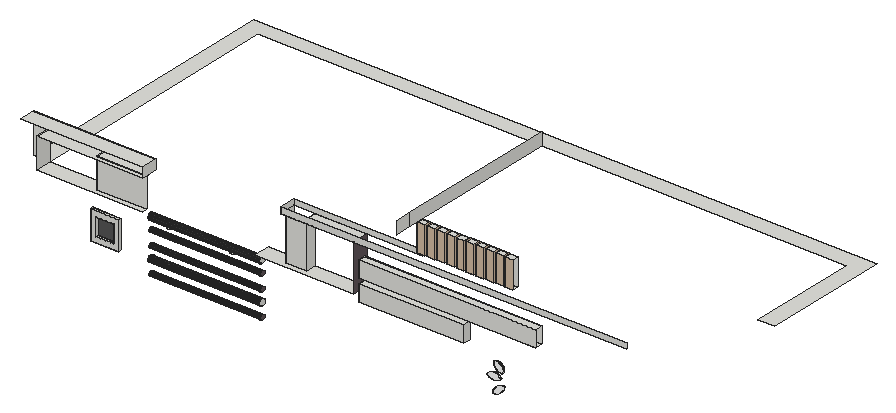
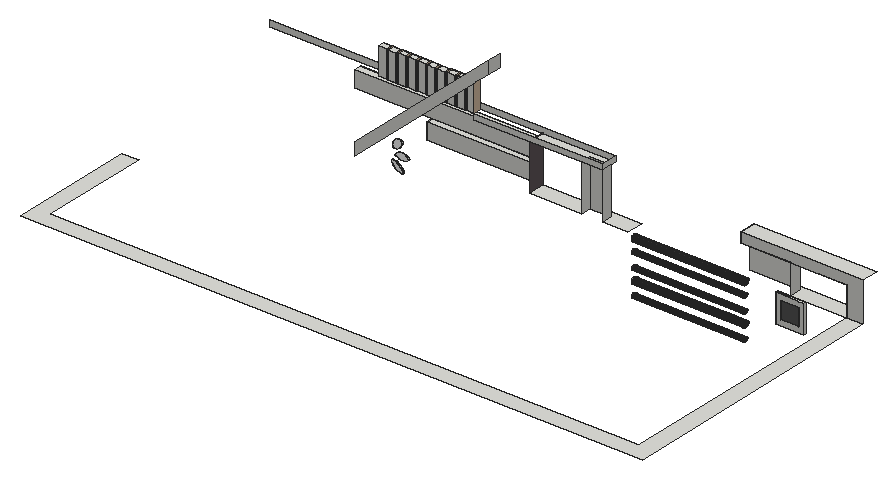
# SketchUp Ruby script. Lengths in inches.
U = 1.inch
M = Sketchup.active_model
def pt(a) = Geom::Point3d.new(a.map { |v| v * U })
def face(e, loops, mat)
  f = e.add_face(loops[0].map { |a| pt(a) })
  loops[1..].each { |l| e.add_face(l.map { |a| pt(a) }).erase! }
  f.material = f.back_material = mat if mat
  f
end
# faces: each face lists its corners as indices into pts; further lists are holes
def faces(e, pts, list, mat = nil) = list.each { |f| face(e, (f[0].is_a?(Array) ? f : [f]).map { |l| l.map { |i| pts[i] } }, mat) }
# xy, xz, yz: faces in a plane at the given z, y or x. An outline is a flat list of corners, or four numbers for a rectangle; further outlines are holes
def ring(l) = l.size == 4 ? [[l[0], l[1]], [l[2], l[1]], [l[2], l[3]], [l[0], l[3]]] : l.each_slice(2).to_a
def flat(e, list, mat, &to3) = list.each { |f| face(e, (f[0].is_a?(Array) ? f : [f]).map { |l| ring(l).map { |u, v| to3.(u, v) } }, mat) }
def xy(e, z, list, mat = nil) = flat(e, list, mat) { |x, y| [x, y, z] }
def xz(e, y, list, mat = nil) = flat(e, list, mat) { |x, z| [x, y, z] }
def yz(e, x, list, mat = nil) = flat(e, list, mat) { |y, z| [x, y, z] }
def lines(e, pts, list) = list.each { |a, b| e.add_line(pt(pts[a]), pt(pts[b])) }
# prism: a flat outline (further loops are holes) pulled along v
def prism(e, loops, v, mat = nil)
  f = face(e, loops, mat); d = Geom::Vector3d.new(v.map { |x| x * U })
  f.pushpull(f.normal.samedirection?(d) ? d.length : -d.length)
end
def box(e, o, s, mat = nil) = prism(e, [[o, [o[0] + s[0], o[1], o[2]], [o[0] + s[0], o[1] + s[1], o[2]], [o[0], o[1] + s[1], o[2]]]], [0, 0, s[2]], mat)
def at(x, y, z, deg = 0) = Geom::Transformation.translation(pt([x, y, z])) * Geom::Transformation.rotation(ORIGIN, Z_AXIS, deg.degrees)
def axes(o, x, y, z) = Geom::Transformation.new([*x, 0, *y, 0, *z, 0, *pt(o).to_a, 1])
def part(name) = M.definitions.add(name)
# library, detail: a bought-in or finely detailed component or shape, given as its bounding box
def library(name, o, s) = part(name).tap { |d| box(d.entities, o, s) }
def detail(e, o, s) = box(e.add_group.entities, o, s)
def put(e, d, t, mat = nil) = e.add_instance(d, t).tap { |i| i.material = mat if mat }
def group(e, t, mat = nil) = e.add_group.tap { |g| g.transformation = t; g.material = mat if mat }.entities
root = M.entities
M.materials.add("[Asphalt New]").color = [96, 86, 89]
M.materials.add("[Color M00]").color = [255, 255, 255]
M.materials.add("[Color M06]").color = [86, 86, 86]
M.materials.add("[Color M07]").color = [58, 58, 58]
M.materials.add("[Formica Laminate Light]").color = [213, 189, 164]
box(root,[255.42,148.16,262.6875],[57.81,4.19,8.9375])
prism(root,[[[323.7,152.35,248.91],[323.08,152.35,249.43],[323.52,152.35,249.97],[324.07,152.35,250.4375],[324.71,152.35,250.82],[325.41,152.35,251.1],[326.17,152.35,251.27],[326.94,152.35,251.33],[327.72,152.35,251.27],[328.47,152.35,251.1],[329.18,152.35,250.82],[329.8125,152.35,250.4375],[330.36,152.35,249.97],[330.81,152.35,249.43],[330.18,152.35,248.91],[329.46,152.35,248.49],[328.66,152.35,248.18],[327.82,152.35,247.99],[326.94,152.35,247.92],[326.07,152.35,247.99],[325.22,152.35,248.18],[324.43,152.35,248.49]]],[0,-0.5625,0],"[Color M00]")
xy(root,239.3,[[105.86,150.85,121.54,152.35]])
xy(root,242.21,[[108.76,150.85,118.64,152.35]])
xy(root,252.08,[[108.76,150.85,118.64,152.35]])
xy(root,254.99,[[105.86,150.85,121.54,152.35]])
xy(root,257.37,[[145.55,154.65,145.96,154.7,146.33,154.86,146.66,155.11,146.9,155.43,147.0625,155.81,147.08,155.94,144.02,155.94,144.04,155.81,144.2,155.43,144.45,155.11,144.77,154.86,145.15,154.7],[180.11,154.65,180.52,154.7,180.9,154.86,181.22,155.11,181.47,155.43,181.625,155.81,181.64,155.94,178.59,155.94,178.6,155.81,178.76,155.43,179.01,155.11,179.33,154.86,179.71,154.7],[144.02,155.94,147.08,155.94,147.11,156.21,147.0625,156.62,146.9,156.99,146.66,157.32,146.33,157.57,145.96,157.72,145.55,157.77,145.15,157.72,144.77,157.57,144.45,157.32,144.2,156.99,144.04,156.62,143.99,156.21],[178.59,155.94,181.64,155.94,181.68,156.21,181.625,156.62,181.47,156.99,181.22,157.32,180.9,157.57,180.52,157.72,180.11,157.77,179.71,157.72,179.33,157.57,179.01,157.32,178.76,156.99,178.6,156.62,178.55,156.21]])
xy(root,262.6875,[[74.99,152.35,133.58,152.35,133.58,154.79,106.04,154.79,106.04,161.35,74.99,161.35],[195.29,152.35,249.72,152.35,249.72,161.35,220.78,161.35,220.78,155.66,209.34,155.66,209.34,161.35,195.29,161.35],[65.99,161.35,74.99,161.35,74.99,304.28,399.27,304.28,399.27,243.33,408.27,243.33,408.27,313.28,65.99,313.28]])
xy(root,274.4,[[255.42,148.16,353.17,152.35]])
xy(root,279.1,[[74.99,152.35,133.58,161.35]])
xy(root,279.1875,[[106.04,154.79,133.58,161.35]])
xy(root,283.34,[[255.42,148.16,353.17,152.35]])
xy(root,284.4375,[[65.99,152.35,133.58,161.35]])
xy(root,288.3125,[[209.34,152.35,209.34,155.66,220.78,155.66,220.78,161.35,249.72,161.35,249.72,152.35]])
xy(root,291.4375,[[280.02,157.85,284.38,161.35],[285.39,157.85,289.76,161.35],[290.77,157.85,295.13,161.35],[296.14,157.85,300.51,161.35],[301.52,157.85,305.88,161.35],
  [306.89,157.85,311.26,161.35],[312.27,157.85,316.63,161.35],[317.64,157.85,322.01,161.35],[323.02,157.85,327.38,161.35],[328.39,157.85,332.76,161.35]])
xy(root,306.375,[[280.02,157.85,284.38,161.35],[285.39,157.85,289.76,161.35],[290.77,157.85,295.13,161.35],[296.14,157.85,300.51,161.35],[301.52,157.85,305.88,161.35],
  [306.89,157.85,311.26,161.35],[312.27,157.85,316.63,161.35],[317.64,157.85,322.01,161.35],[323.02,157.85,327.38,161.35],[328.39,157.85,332.76,161.35]])
xz(root,148.16,[[255.42,274.4,353.17,283.34]])
xz(root,150.85,[[[105.86,239.3,121.54,254.99],[108.76,242.21,118.64,252.08]]])
xz(root,151.79,[[326.99,241.29,327.73,241.32,328.46,241.46,329.16,241.68,329.83,242,330.45,242.4,331.01,242.89,331.5,243.4375,331.92,244.05,332.25,244.71,332.5,245.4,332.64,246.13,331.92,246.15,331.19,246.09,330.48,245.93,329.79,245.69,329.14,245.37,328.53,244.97,327.97,244.5,327.48,243.96,327.05,243.37,326.7,242.73,326.4375,242.06,326.25,241.35],[331.37,252.53,332.01,252.625,332.1875,253.33,332.22,254.0625,332.1,254.78,331.84,255.47,331.45,256.08,330.9375,256.6,330.33,257.01,329.66,257.29,328.94,257.43,328.21,257.42,327.5,257.27,326.83,256.97,326.85,256.32,326.97,255.68,327.1875,255.07,327.5,254.5,327.89,253.98,328.35,253.52,328.88,253.14,329.46,252.85,330.08,252.65,330.72,252.54]],"[Color M00]")
xz(root,152.35,[[[105.86,239.3,121.54,254.99],[108.76,242.21,118.64,252.08]],[255.42,274.4,353.17,283.34],[209.34,288.3125,399.65,291.4375]])
xz(root,152.35,[[326.99,241.29,326.25,241.35,326.4375,242.06,326.7,242.73,327.05,243.37,327.48,243.96,327.97,244.5,328.53,244.97,329.14,245.37,329.79,245.69,330.48,245.93,331.19,246.09,331.92,246.15,332.64,246.13,332.5,245.4,332.25,244.71,331.92,244.05,331.5,243.4375,331.01,242.89,330.45,242.4,329.83,242,329.16,241.68,328.46,241.46,327.73,241.32],[331.37,252.53,330.72,252.54,330.08,252.65,329.46,252.85,328.88,253.14,328.35,253.52,327.89,253.98,327.5,254.5,327.1875,255.07,326.97,255.68,326.85,256.32,326.83,256.97,327.5,257.27,328.21,257.42,328.94,257.43,329.66,257.29,330.33,257.01,330.9375,256.6,331.45,256.08,331.84,255.47,332.1,254.78,332.22,254.0625,332.1875,253.33,332.01,252.625]],"[Color M00]")
xz(root,152.35,[[108.76,242.21,118.64,252.08]],"[Color M06]")
xz(root,154.79,[[106.04,262.6875,133.58,279.1875]])
xz(root,155.66,[[209.34,262.6875,220.78,288.3125]])
xz(root,157.85,[[280.02,291.4375,284.38,306.375],[285.39,291.4375,289.76,306.375],[290.77,291.4375,295.13,306.375],[296.14,291.4375,300.51,306.375],[301.52,291.4375,305.88,306.375],
  [306.89,291.4375,311.26,306.375],[312.27,291.4375,316.63,306.375],[317.64,291.4375,322.01,306.375],[323.02,291.4375,327.38,306.375],[328.39,291.4375,332.76,306.375]],"[Formica Laminate Light]")
xz(root,161.35,[[65.99,262.6875,65.99,284.4375,133.58,284.4375,133.58,279.1875,106.04,279.1875,106.04,279.1,74.99,279.1,74.99,262.6875],[106.04,279.1,133.58,279.1875],[209.34,288.3125,280.02,291.4375],[280.02,291.4375,284.38,306.375],[284.38,291.4375,285.39,306.375],
  [285.39,291.4375,289.76,306.375],[289.76,291.4375,290.77,306.375],[290.77,291.4375,295.13,306.375],[295.13,291.4375,296.14,306.375],[296.14,291.4375,300.51,306.375],
  [300.51,291.4375,301.52,306.375],[301.52,291.4375,305.88,306.375],[305.88,291.4375,306.89,306.375],[306.89,291.4375,311.26,306.375],[311.26,291.4375,312.27,306.375],
  [312.27,291.4375,316.63,306.375],[316.63,291.4375,317.64,306.375],[317.64,291.4375,322.01,306.375],[322.01,291.4375,323.02,306.375],[323.02,291.4375,327.38,306.375],
  [327.38,291.4375,328.39,306.375],[328.39,291.4375,332.76,306.375]])
yz(root,74.99,[[152.35,262.6875,161.35,279.1]])
yz(root,105.86,[[150.85,239.3,152.35,254.99]])
yz(root,106.04,[[154.79,262.6875,161.35,279.1875]])
yz(root,108.76,[[150.85,242.21,152.35,252.08]])
yz(root,118.64,[[150.85,242.21,152.35,252.08]])
yz(root,121.54,[[150.85,239.3,152.35,254.99]])
yz(root,133.58,[[152.35,279.1,154.79,279.1,154.79,279.1875,161.35,279.1875,161.35,284.4375,152.35,284.4375],[154.79,279.1,161.35,279.1875]])
yz(root,195.29,[[157.4,235.59,157.84,235.65,158.25,235.82,158.6,236.08,158.87,236.43,159.03,236.84,159.09,237.28,159.03,237.71,158.87,238.12,158.6,238.47,158.25,238.74,157.84,238.91,157.4,238.96,156.97,238.91,156.5625,238.74,156.21,238.47,155.94,238.12,155.77,237.71,155.72,237.28,155.77,236.84,155.94,236.43,156.21,236.08,156.5625,235.82,156.97,235.65],[157.4,256.53,157.84,256.58,158.25,256.75,158.6,257.02,158.87,257.37,159.03,257.78,159.09,258.21,159.03,258.65,158.87,259.06,158.6,259.41,158.25,259.68,157.84,259.84,157.4,259.9,156.97,259.84,156.5625,259.68,156.21,259.41,155.94,259.06,155.77,258.65,155.72,258.21,155.77,257.78,155.94,257.37,156.21,257.02,156.5625,256.75,156.97,256.58]])
yz(root,195.29,[[157.64,228.69,157.94,228.73,158.23,228.85,158.48,229.04,158.67,229.28,158.78,229.57,158.82,229.88,158.78,230.1875,158.67,230.47,158.48,230.72,158.23,230.91,157.94,231.03,157.64,231.07,157.33,231.03,157.04,230.91,156.8,230.72,156.61,230.47,156.49,230.1875,156.45,229.88,156.49,229.57,156.61,229.28,156.8,229.04,157.04,228.85,157.33,228.73],[157.64,242.44,157.94,242.48,158.23,242.6,158.48,242.79,158.67,243.03,158.78,243.32,158.82,243.63,158.78,243.9375,158.67,244.22,158.48,244.47,158.23,244.66,157.94,244.78,157.64,244.82,157.33,244.78,157.04,244.66,156.8,244.47,156.61,244.22,156.49,243.9375,156.45,243.63,156.49,243.32,156.61,243.03,156.8,242.79,157.04,242.6,157.33,242.48],[157.64,250.38,157.94,250.42,158.23,250.54,158.48,250.73,158.67,250.97,158.78,251.26,158.82,251.57,158.78,251.875,158.67,252.16,158.48,252.41,158.23,252.59,157.94,252.71,157.64,252.75,157.33,252.71,157.04,252.59,156.8,252.41,156.61,252.16,156.49,251.875,156.45,251.57,156.49,251.26,156.61,250.97,156.8,250.73,157.04,250.54,157.33,250.42]],"[Asphalt New]")
yz(root,209.34,[[155.66,262.6875,161.35,288.3125],[152.35,288.3125,161.35,291.4375]])
yz(root,220.78,[[155.66,262.6875,161.35,288.3125]])
yz(root,249.72,[[152.35,262.6875,161.35,288.3125]],"[Asphalt New]")
yz(root,255.42,[[148.16,274.4,152.35,283.34]])
yz(root,280.02,[[143.85,306.375,152.35,313.1875],[152.35,306.375,243.33,313.1875]])
yz(root,280.02,[[157.85,291.4375,161.35,306.375]],"[Formica Laminate Light]")
yz(root,284.38,[[157.85,291.4375,161.35,306.375]],"[Formica Laminate Light]")
yz(root,285.39,[[157.85,291.4375,161.35,306.375]],"[Formica Laminate Light]")
yz(root,289.76,[[157.85,291.4375,161.35,306.375]],"[Formica Laminate Light]")
yz(root,290.77,[[157.85,291.4375,161.35,306.375]],"[Formica Laminate Light]")
yz(root,295.13,[[157.85,291.4375,161.35,306.375]],"[Formica Laminate Light]")
yz(root,296.14,[[157.85,291.4375,161.35,306.375]],"[Formica Laminate Light]")
yz(root,300.51,[[157.85,291.4375,161.35,306.375]],"[Formica Laminate Light]")
yz(root,301.52,[[157.85,291.4375,161.35,306.375]],"[Formica Laminate Light]")
yz(root,305.88,[[157.85,291.4375,161.35,306.375]],"[Formica Laminate Light]")
yz(root,306.89,[[157.85,291.4375,161.35,306.375]],"[Formica Laminate Light]")
yz(root,311.26,[[157.85,291.4375,161.35,306.375]],"[Formica Laminate Light]")
yz(root,312.27,[[157.85,291.4375,161.35,306.375]],"[Formica Laminate Light]")
yz(root,316.63,[[157.85,291.4375,161.35,306.375]],"[Formica Laminate Light]")
yz(root,317.64,[[157.85,291.4375,161.35,306.375]],"[Formica Laminate Light]")
yz(root,322.01,[[157.85,291.4375,161.35,306.375]],"[Formica Laminate Light]")
yz(root,323.02,[[157.85,291.4375,161.35,306.375]],"[Formica Laminate Light]")
yz(root,327.38,[[157.85,291.4375,161.35,306.375]],"[Formica Laminate Light]")
yz(root,328.39,[[157.85,291.4375,161.35,306.375]],"[Formica Laminate Light]")
p = [[195.29,157.33,228.73],[195.29,157.04,228.85],[133.58,157.04,228.85],[133.58,157.33,228.73],[195.29,157.64,228.69],[133.58,157.64,228.69],
  [195.29,157.94,228.73],[133.58,157.94,228.73],[195.29,158.23,228.85],[133.58,158.23,228.85],[195.29,156.8,229.04],[133.58,156.8,229.04],
  [195.29,158.48,229.04],[133.58,158.48,229.04],[195.29,156.61,229.28],[133.58,156.61,229.28],[195.29,158.67,229.28],[133.58,158.67,229.28],
  [195.29,156.49,229.57],[133.58,156.49,229.57],[195.29,158.78,229.57],[133.58,158.78,229.57],[195.29,156.45,229.88],[133.58,156.45,229.88],
  [195.29,158.82,229.88],[133.58,158.82,229.88],[195.29,156.49,230.1875],[133.58,156.49,230.1875],[195.29,158.78,230.1875],[133.58,158.78,230.1875],
  [195.29,156.61,230.47],[133.58,156.61,230.47],[195.29,158.67,230.47],[133.58,158.67,230.47],[195.29,156.8,230.72],[133.58,156.8,230.72],
  [195.29,158.48,230.72],[133.58,158.48,230.72],[195.29,157.04,230.91],[133.58,157.04,230.91],[195.29,158.23,230.91],[133.58,158.23,230.91],
  [195.29,157.33,231.03],[133.58,157.33,231.03],[195.29,157.94,231.03],[133.58,157.94,231.03],[195.29,157.64,231.07],[133.58,157.64,231.07],
  [195.29,156.97,235.65],[195.29,156.5625,235.82],[133.58,156.5625,235.82],[133.58,156.97,235.65],[195.29,157.4,235.59],[133.58,157.4,235.59],
  [195.29,157.84,235.65],[133.58,157.84,235.65],[195.29,158.25,235.82],[133.58,158.25,235.82],[195.29,156.21,236.08],[181.68,156.21,236.08],
  [178.55,156.21,236.08],[147.11,156.21,236.08],[143.99,156.21,236.08],[133.58,156.21,236.08],[195.29,158.6,236.08],[133.58,158.6,236.08],
  [195.29,155.94,236.43],[133.58,155.94,236.43],[195.29,158.87,236.43],[133.58,158.87,236.43],[195.29,155.77,236.84],[133.58,155.77,236.84],
  [195.29,159.03,236.84],[133.58,159.03,236.84],[195.29,155.72,237.28],[133.58,155.72,237.28],[195.29,159.09,237.28],[133.58,159.09,237.28],
  [195.29,155.77,237.71],[133.58,155.77,237.71],[195.29,159.03,237.71],[133.58,159.03,237.71],[195.29,155.94,238.12],[133.58,155.94,238.12],
  [195.29,158.87,238.12],[133.58,158.87,238.12],[195.29,156.21,238.47],[181.68,156.21,238.47],[178.55,156.21,238.47],[147.11,156.21,238.47],
  [143.99,156.21,238.47],[133.58,156.21,238.47],[195.29,158.6,238.47],[133.58,158.6,238.47],[195.29,156.5625,238.74],[133.58,156.5625,238.74],
  [195.29,158.25,238.74],[133.58,158.25,238.74],[195.29,156.97,238.91],[133.58,156.97,238.91],[195.29,157.84,238.91],[133.58,157.84,238.91],
  [195.29,157.4,238.96],[133.58,157.4,238.96],[326.4375,152.35,242.06],[326.25,152.35,241.35],[326.25,151.79,241.35],[326.4375,151.79,242.06],
  [326.99,152.35,241.29],[326.99,151.79,241.29],[327.73,152.35,241.32],[327.73,151.79,241.32],[328.46,152.35,241.46],[328.46,151.79,241.46],
  [329.16,152.35,241.68],[329.16,151.79,241.68],[329.83,152.35,242],[329.83,151.79,242],[330.45,152.35,242.4],[330.45,151.79,242.4],
  [326.7,152.35,242.73],[326.7,151.79,242.73],[331.01,152.35,242.89],[331.01,151.79,242.89],[195.29,157.64,242.44],[195.29,157.33,242.48],
  [133.58,157.33,242.48],[133.58,157.64,242.44],[195.29,157.94,242.48],[133.58,157.94,242.48],[195.29,157.04,242.6],[133.58,157.04,242.6],
  [195.29,158.23,242.6],[133.58,158.23,242.6],[195.29,156.8,242.79],[133.58,156.8,242.79],[195.29,158.48,242.79],[133.58,158.48,242.79],
  [327.05,152.35,243.37],[327.05,151.79,243.37],[195.29,156.61,243.03],[133.58,156.61,243.03],[195.29,158.67,243.03],[133.58,158.67,243.03],
  [331.5,152.35,243.4375],[331.5,151.79,243.4375],[195.29,156.49,243.32],[133.58,156.49,243.32],[195.29,158.78,243.32],[133.58,158.78,243.32],
  [195.29,156.45,243.63],[133.58,156.45,243.63],[195.29,158.82,243.63],[133.58,158.82,243.63],[327.48,152.35,243.96],[327.48,151.79,243.96],
  [331.92,152.35,244.05],[331.92,151.79,244.05],[195.29,156.49,243.9375],[133.58,156.49,243.9375],[195.29,158.78,243.9375],[133.58,158.78,243.9375],
  [195.29,156.61,244.22],[133.58,156.61,244.22],[195.29,158.67,244.22],[133.58,158.67,244.22],[327.97,152.35,244.5],[327.97,151.79,244.5],
  [332.25,152.35,244.71],[332.25,151.79,244.71],[195.29,156.8,244.47],[133.58,156.8,244.47],[195.29,158.48,244.47],[133.58,158.48,244.47],
  [328.53,152.35,244.97],[328.53,151.79,244.97],[195.29,157.04,244.66],[133.58,157.04,244.66],[195.29,158.23,244.66],[133.58,158.23,244.66],
  [195.29,157.33,244.78],[133.58,157.33,244.78],[195.29,157.94,244.78],[133.58,157.94,244.78],[195.29,157.64,244.82],[133.58,157.64,244.82],
  [329.14,152.35,245.37],[329.14,151.79,245.37],[329.79,152.35,245.69],[329.79,151.79,245.69],[330.48,152.35,245.93],[330.48,151.79,245.93],
  [331.19,152.35,246.09],[331.19,151.79,246.09],[331.92,152.35,246.15],[331.92,151.79,246.15],[195.29,157.33,250.42],[195.29,157.04,250.54],
  [133.58,157.04,250.54],[133.58,157.33,250.42],[195.29,157.64,250.38],[133.58,157.64,250.38],[195.29,157.94,250.42],[133.58,157.94,250.42],
  [195.29,158.23,250.54],[133.58,158.23,250.54],[195.29,156.8,250.73],[133.58,156.8,250.73],[195.29,158.48,250.73],[133.58,158.48,250.73],
  [195.29,156.61,250.97],[133.58,156.61,250.97],[195.29,158.67,250.97],[133.58,158.67,250.97],[195.29,156.49,251.26],[133.58,156.49,251.26],
  [195.29,158.78,251.26],[133.58,158.78,251.26],[195.29,156.45,251.57],[133.58,156.45,251.57],[195.29,158.82,251.57],[133.58,158.82,251.57],
  [195.29,156.49,251.875],[133.58,156.49,251.875],[195.29,158.78,251.875],[133.58,158.78,251.875],[195.29,156.61,252.16],[133.58,156.61,252.16],
  [195.29,158.67,252.16],[133.58,158.67,252.16],[195.29,156.8,252.41],[133.58,156.8,252.41],[195.29,158.48,252.41],[133.58,158.48,252.41],
  [195.29,157.04,252.59],[133.58,157.04,252.59],[195.29,158.23,252.59],[133.58,158.23,252.59],[330.08,152.35,252.65],[330.72,152.35,252.54],
  [330.72,151.79,252.54],[330.08,151.79,252.65],[331.37,152.35,252.53],[331.37,151.79,252.53],[332.01,152.35,252.625],[332.01,151.79,252.625],
  [329.46,152.35,252.85],[329.46,151.79,252.85],[332.1875,152.35,253.33],[332.1875,151.79,253.33],[195.29,157.33,252.71],[133.58,157.33,252.71],
  [195.29,157.94,252.71],[133.58,157.94,252.71],[195.29,157.64,252.75],[133.58,157.64,252.75],[328.88,152.35,253.14],[328.88,151.79,253.14],
  [328.35,152.35,253.52],[328.35,151.79,253.52],[327.89,152.35,253.98],[327.89,151.79,253.98],[327.5,152.35,254.5],[327.5,151.79,254.5],
  [332.22,152.35,254.0625],[332.1,152.35,254.78],[332.1,151.79,254.78],[332.22,151.79,254.0625],[327.1875,152.35,255.07],[327.1875,151.79,255.07],
  [331.84,152.35,255.47],[331.84,151.79,255.47],[326.97,152.35,255.68],[326.97,151.79,255.68],[331.45,152.35,256.08],[331.45,151.79,256.08],
  [326.85,152.35,256.32],[326.85,151.79,256.32],[330.9375,152.35,256.6],[330.9375,151.79,256.6],[326.83,152.35,256.97],[326.83,151.79,256.97],
  [195.29,157.4,256.53],[195.29,156.97,256.58],[133.58,156.97,256.58],[133.58,157.4,256.53],[195.29,157.84,256.58],[133.58,157.84,256.58],
  [330.33,152.35,257.01],[330.33,151.79,257.01],[195.29,156.5625,256.75],[133.58,156.5625,256.75],[195.29,158.25,256.75],[133.58,158.25,256.75],
  [195.29,156.21,257.02],[181.68,156.21,257.02],[178.55,156.21,257.02],[147.11,156.21,257.02],[143.99,156.21,257.02],[133.58,156.21,257.02],
  [195.29,158.6,257.02],[133.58,158.6,257.02],[327.5,152.35,257.27],[327.5,151.79,257.27],[329.66,152.35,257.29],[329.66,151.79,257.29],
  [195.29,155.94,257.37],[181.64,155.94,257.37],[178.59,155.94,257.37],[147.08,155.94,257.37],[144.02,155.94,257.37],[133.58,155.94,257.37],
  [195.29,158.87,257.37],[133.58,158.87,257.37],[328.21,152.35,257.42],[328.21,151.79,257.42],[328.94,152.35,257.43],[328.94,151.79,257.43],
  [195.29,155.77,257.78],[133.58,155.77,257.78],[195.29,159.03,257.78],[133.58,159.03,257.78],[195.29,155.72,258.21],[133.58,155.72,258.21],
  [195.29,159.09,258.21],[133.58,159.09,258.21],[195.29,155.77,258.65],[133.58,155.77,258.65],[195.29,159.03,258.65],[133.58,159.03,258.65],
  [195.29,155.94,259.06],[133.58,155.94,259.06],[195.29,158.87,259.06],[133.58,158.87,259.06],[195.29,156.21,259.41],[133.58,156.21,259.41],
  [195.29,158.6,259.41],[133.58,158.6,259.41],[195.29,156.5625,259.68],[133.58,156.5625,259.68],[195.29,158.25,259.68],[133.58,158.25,259.68],
  [195.29,156.97,259.84],[133.58,156.97,259.84],[195.29,157.84,259.84],[133.58,157.84,259.84],[195.29,157.4,259.9],[133.58,157.4,259.9]]
faces(root,p,[[0,1,2,3],[4,0,3,5],[6,4,5,7],[8,6,7,9],[1,10,11,2],[12,8,9,13],[10,14,15,11],[16,12,13,17],
  [14,18,19,15],[20,16,17,21],[18,22,23,19],[24,20,21,25],[22,26,27,23],[28,24,25,29],[26,30,31,27],[32,28,29,33],
  [30,34,35,31],[36,32,33,37],[34,38,39,35],[40,36,37,41],[38,42,43,39],[44,40,41,45],[42,46,47,43],[46,44,45,47],
  [48,49,50,51],[52,48,51,53],[54,52,53,55],[56,54,55,57],[49,58,59,60,61,62,63,50],[64,56,57,65],[58,66,67,63,62,61,60,59],[68,64,65,69],
  [66,70,71,67],[72,68,69,73],[70,74,75,71],[76,72,73,77],[74,78,79,75],[80,76,77,81],[78,82,83,79],[84,80,81,85],
  [82,86,87,88,89,90,91,83],[92,84,85,93],[86,94,95,91,90,89,88,87],[96,92,93,97],[94,98,99,95],[100,96,97,101],[98,102,103,99],[102,100,101,103],
  [124,125,126,127],[128,124,127,129],[125,130,131,126],[132,128,129,133],[130,134,135,131],[136,132,133,137],[134,140,141,135],[142,136,137,143],
  [140,146,147,141],[148,142,143,149],[146,150,151,147],[152,148,149,153],[150,158,159,151],[160,152,153,161],[158,162,163,159],[164,160,161,165],
  [162,170,171,163],[172,164,165,173],[170,176,177,171],[178,172,173,179],[176,180,181,177],[182,178,179,183],[180,184,185,181],[184,182,183,185],
  [196,197,198,199],[200,196,199,201],[202,200,201,203],[204,202,203,205],[197,206,207,198],[208,204,205,209],[206,210,211,207],[212,208,209,213],
  [210,214,215,211],[216,212,213,217],[214,218,219,215],[220,216,217,221],[218,222,223,219],[224,220,221,225],[222,226,227,223],[228,224,225,229],
  [226,230,231,227],[232,228,229,233],[230,234,235,231],[236,232,233,237],[234,250,251,235],[252,236,237,253],[250,254,255,251],[254,252,253,255],
  [282,283,284,285],[286,282,285,287],[283,290,291,284],[292,286,287,293],[290,294,295,296,297,298,299,291],[300,292,293,301],[294,306,307,308,309,310,311,299,298,297,296,295],[312,300,301,313],
  [306,318,319,311,310,309,308,307],[320,312,313,321],[318,322,323,319],[324,320,321,325],[322,326,327,323],[328,324,325,329],[326,330,331,327],[332,328,329,333],
  [330,334,335,331],[336,332,333,337],[334,338,339,335],[340,336,337,341],[338,342,343,339],[344,340,341,345],[342,346,347,343],[346,344,345,347]],"[Color M07]")
faces(root,p,[[104,105,106,107],[105,108,109,106],[108,110,111,109],[110,112,113,111],[112,114,115,113],[114,116,117,115],[116,118,119,117],[120,104,107,121],
  [118,122,123,119],[138,120,121,139],[122,144,145,123],[154,138,139,155],[144,156,157,145],[166,154,155,167],[156,168,169,157],[174,166,167,175],
  [186,174,175,187],[188,186,187,189],[190,188,189,191],[192,190,191,193],[194,192,193,195],[238,239,240,241],[239,242,243,240],[242,244,245,243],
  [246,238,241,247],[244,248,249,245],[256,246,247,257],[258,256,257,259],[260,258,259,261],[262,260,261,263],[264,265,266,267],[268,262,263,269],
  [265,270,271,266],[272,268,269,273],[270,274,275,271],[276,272,273,277],[274,278,279,275],[280,276,277,281],[278,288,289,279],[302,280,281,303],
  [288,304,305,289],[314,302,303,315],[304,316,317,305],[316,314,315,317]],"[Color M00]")
